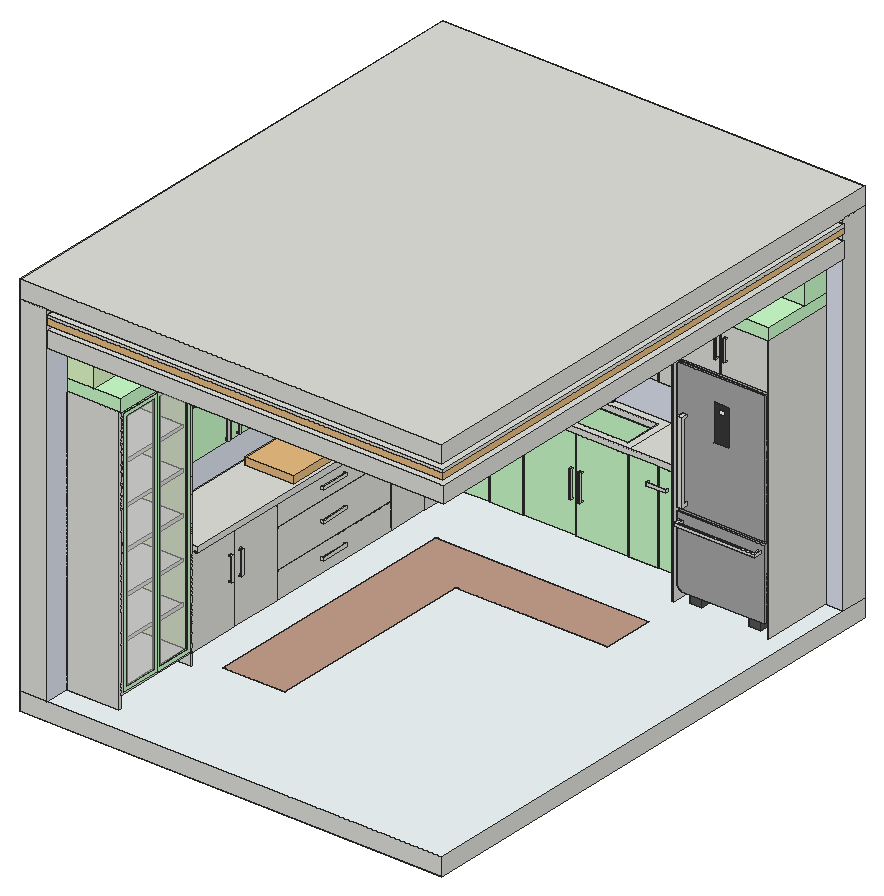
# SketchUp Ruby script. Lengths in inches.
U = 1.inch
M = Sketchup.active_model
def pt(a) = Geom::Point3d.new(a.map { |v| v * U })
def face(e, loops, mat)
  f = e.add_face(loops[0].map { |a| pt(a) })
  loops[1..].each { |l| e.add_face(l.map { |a| pt(a) }).erase! }
  f.material = f.back_material = mat if mat
  f
end
# faces: each face lists its corners as indices into pts; further lists are holes
def faces(e, pts, list, mat = nil) = list.each { |f| face(e, (f[0].is_a?(Array) ? f : [f]).map { |l| l.map { |i| pts[i] } }, mat) }
# xy, xz, yz: faces in a plane at the given z, y or x. An outline is a flat list of corners, or four numbers for a rectangle; further outlines are holes
def ring(l) = l.size == 4 ? [[l[0], l[1]], [l[2], l[1]], [l[2], l[3]], [l[0], l[3]]] : l.each_slice(2).to_a
def flat(e, list, mat, &to3) = list.each { |f| face(e, (f[0].is_a?(Array) ? f : [f]).map { |l| ring(l).map { |u, v| to3.(u, v) } }, mat) }
def xy(e, z, list, mat = nil) = flat(e, list, mat) { |x, y| [x, y, z] }
def xz(e, y, list, mat = nil) = flat(e, list, mat) { |x, z| [x, y, z] }
def yz(e, x, list, mat = nil) = flat(e, list, mat) { |y, z| [x, y, z] }
def lines(e, pts, list) = list.each { |a, b| e.add_line(pt(pts[a]), pt(pts[b])) }
# prism: a flat outline (further loops are holes) pulled along v
def prism(e, loops, v, mat = nil)
  f = face(e, loops, mat); d = Geom::Vector3d.new(v.map { |x| x * U })
  f.pushpull(f.normal.samedirection?(d) ? d.length : -d.length)
end
def box(e, o, s, mat = nil) = prism(e, [[o, [o[0] + s[0], o[1], o[2]], [o[0] + s[0], o[1] + s[1], o[2]], [o[0], o[1] + s[1], o[2]]]], [0, 0, s[2]], mat)
def at(x, y, z, deg = 0) = Geom::Transformation.translation(pt([x, y, z])) * Geom::Transformation.rotation(ORIGIN, Z_AXIS, deg.degrees)
def axes(o, x, y, z) = Geom::Transformation.new([*x, 0, *y, 0, *z, 0, *pt(o).to_a, 1])
def part(name) = M.definitions.add(name)
# library, detail: a bought-in or finely detailed component or shape, given as its bounding box
def library(name, o, s) = part(name).tap { |d| box(d.entities, o, s) }
def detail(e, o, s) = box(e.add_group.entities, o, s)
def put(e, d, t, mat = nil) = e.add_instance(d, t).tap { |i| i.material = mat if mat }
def group(e, t, mat = nil) = e.add_group.tap { |g| g.transformation = t; g.material = mat if mat }.entities
root = M.entities
M.materials.add("[Color E01]").color = [255, 255, 204]
M.materials.add("[Color E04]").color = [255, 255, 50]
M.materials.add("[Color E05]").color = [255, 255, 0]
M.materials.add("[Color F01]").color = [229, 255, 204]
M.materials.add("[Color G01]").color = [204, 255, 204]
M.materials.add("[Color M00]").color = [255, 255, 255]
M.materials.add("[Color M03]").color = [170, 170, 170]
M.materials.add("[Color M06]").color = [86, 86, 86]
M.materials.add("[Color M07]").color = [58, 58, 58]
M.materials.add("[Color M08]").color = [30, 30, 30]
M.materials.add("[Color M09]").color = [0, 0, 0]
M.materials.add("[Marble Carrara Floor Tile]").color = [225, 230, 242]
M.materials.add("[Translucent Glass Gray]").color = [232, 232, 232]
M.materials["[Translucent Glass Gray]"].alpha = 0.5
M.materials.add("[Translucent Glass Gray]1").color = [219, 219, 219]
M.materials["[Translucent Glass Gray]1"].alpha = 0.5
M.materials.add("[Upholstery Striped Multi-Colored]").color = [198, 159, 140]
M.materials.add("[White Subway Tile]").color = [243, 252, 253]
c1 = part("Group\#6")
box(c1.entities,[0,0,0],[17,26,1])
c2 = library("Group\#43",[0,0,0],[16.5,36,2.3125])
c3 = part("Group\#46")
prism(c3.entities,[[[0,1,0],[0,1,0.4],[0.8,1,0.4],[0.8,1,9.6],[0,1,9.6],[0,1,10],[1.2,1,10],[1.2,1,0]]],[0,-1,0])
c4 = part("Group\#47")
prism(c4.entities,[[[0,0,6.4375],[0,0,6.1],[0.66,0,6.1],[0.66,0,0.34],[0,0,0.34],[0,0,0],[1,0,0],[1,0,6.4375]]],[0,0.6875,0])
c5 = part("Group\#49")
prism(c5.entities,[[[0.875,0.31,9],[0.875,1,9],[0.875,1,9.3125],[0.875,0,9.3125],[0.875,0,0],[0.875,1,0],[0.875,1,0.31],[0.875,0.31,0.31]]],[-0.875,0,0])
c6 = part("Group\#50")
prism(c6.entities,[[[6.64,1,0],[6.9375,1,0],[6.9375,0,0],[0,0,0],[0,1,0],[0.3,1,0],[0.3,0.3,0],[6.64,0.3,0]]],[0,0,0.9375])
c7 = part("Group\#51")
prism(c7.entities,[[[0.6875,1,6.95],[0.6875,1,7.25],[0.6875,0,7.25],[0.6875,0,0],[0.6875,1,0],[0.6875,1,0.3],[0.6875,0.3,0.3],[0.6875,0.3,6.95]]],[-0.6875,0,0])
c8 = part("Group\#52")
prism(c8.entities,[[[0,0.5,0],[0,0.5,0.29],[0.8,0.5,0.29],[0.8,0.5,6.98],[0,0.5,6.98],[0,0.5,7.28],[1.2,0.5,7.28],[1.2,0.5,0]]],[0,-0.5,0])
c9 = library("Group\#56",[0,0,0],[135,171,2])
c10 = part("Group\#63")
detail(c10.entities,[0,0,0],[2,2,1.9375])
box(root,[24.44,95.55,73.22],[0.1,9.82,0.69])
xy(root,6,[[34.24,44.3,34.24,134.73,107.05,134.73,107.05,117.05,55.37,117.05,55.37,44.3]])
xy(root,6.01,[[34.24,44.3,55.37,44.3,55.37,117.05,107.05,117.05,107.05,134.73,34.24,134.73]],"[Upholstery Striped Multi-Colored]")
xz(root,44.3,[[34.24,6,55.37,6.01]])
xz(root,117.05,[[55.37,6,107.05,6.01]])
xz(root,134.73,[[34.24,6,107.05,6.01]])
xz(root,147.3,[[121.27,68.89,122.52,70.08]],"[Color M00]")
xz(root,152.9,[[50.8,68.5,66.65,83.5],[67.65,68.5,83.5,83.5]],"[Translucent Glass Gray]")
yz(root,27.5,[[11.5,12.1,23.5,95.05]],"[Translucent Glass Gray]")
yz(root,34.24,[[44.3,6,134.73,6.01]])
yz(root,55.37,[[44.3,6,117.05,6.01]])
yz(root,107.05,[[117.05,6,134.73,6.01]])
p = [[27.5,25.5,95.05],[27,37.5,95.05],[27,37.5,12.1],[27.5,25.5,12.1],[25,106.3,84],[25,94.3,84],
  [10,94.3,84],[10,106.3,84],[11,100.6,45],[27,100.6,45]]
faces(root,p,[[0,1,2,3]],"[Translucent Glass Gray]1")
lines(root,p,[[4,5],[5,6],[6,7],[7,4],[8,9]])
g1 = group(root,at(0,84.5,0))
xy(g1,0,[[0,-84,144,96]])
xy(g1,6,[[0,-84,144,96]],"[White Subway Tile]")
xz(g1,-84,[[0,0,144,6]])
xz(g1,96,[[0,0,144,6]])
yz(g1,0,[[-84,0,96,6]])
yz(g1,144,[[-84,0,96,6]])
g2 = group(root,at(9,171.5,6))
xy(g2,0,[[0,0,135,9]])
xy(g2,120,[[0,0,135,9]])
xz(g2,0,[[0,0,135,120]],"[Marble Carrara Floor Tile]")
xz(g2,9,[[0,0,135,120]])
yz(g2,0,[[0,0,9,120]])
yz(g2,135,[[0,0,9,120]])
g3 = group(root,at(0,84.5,6))
xy(g3,0,[[0,-84,9,96]])
xy(g3,120,[[0,-84,9,96]])
xz(g3,-84,[[0,0,9,120]])
xz(g3,96,[[0,0,9,120]])
yz(g3,0,[[-84,0,96,120]])
yz(g3,9,[[-84,0,96,120]],"[Marble Carrara Floor Tile]")
g4 = group(root,at(9,9.5,6),"[Color G01]")
box(g4,[0,30.5,0],[10,131.5,4])
g5 = group(root,at(9,39.5,6))
box(g5,[0,0,0],[18,0.5,91.15])
g6 = group(root,at(9,9.5,6),"[Color G01]")
box(g6,[0,0,0],[12,30,4])
g7 = group(root,at(9,9,6))
box(g7,[0,0,0],[18,0.5,91.15])
g8 = group(root,at(9,40,10))
xy(g8,0,[[0,0,0,36,18,36,18,18.15,17.7,18.15,17.7,17.85,18,17.85,18,0],[0,36,18,36.6],[0,36.6,18,84.6],[0,84.6,18,84.9],[0,84.9,0,131.5,18,131.5,18,99.5,17.7,99.5,17.7,98.9,18,98.9,18,84.9]])
xy(g8,9,[[14.4,36.6,18,84.6]])
xy(g8,9.3,[[14.4,36.6,18,84.6]])
xy(g8,22,[[14.4,36.6,18,84.6]])
xy(g8,22.3,[[14.4,36.6,18,84.6]])
xy(g8,31,[[0,0,18,0,18,17.85,17.7,17.85,17.7,18.15,18,18.15,18,36,0,36],[0,36,18,36.6],[0,36.6,18,84.6],[0,84.6,18,84.9],[0,84.9,18,84.9,18,98.9,17.7,98.9,17.7,99.5,18,99.5,18,131.5,0,131.5]])
xz(g8,0,[[0,0,18,31]])
xz(g8,17.85,[[17.7,0,18,31]])
xz(g8,18.15,[[17.7,0,18,31]])
xz(g8,36,[[0,0,18,31]])
xz(g8,36.6,[[0,0,0,31,18,31,18,22.3,14.4,22.3,14.4,22,18,22,18,9.3,14.4,9.3,14.4,9,18,9,18,0],[14.4,9,18,9.3],[14.4,22,18,22.3]])
xz(g8,84.6,[[0,0,0,31,18,31,18,22.3,14.4,22.3,14.4,22,18,22,18,9.3,14.4,9.3,14.4,9,18,9,18,0],[14.4,9,18,9.3],[14.4,22,18,22.3]])
xz(g8,84.9,[[0,0,18,31]])
xz(g8,98.9,[[17.7,0,18,31]])
xz(g8,99.5,[[17.7,0,18,31]])
xz(g8,131.5,[[0,0,18,31]])
yz(g8,0,[[0,0,36,31],[36,0,36.6,31],[36.6,0,84.6,31],[84.6,0,84.9,31],[84.9,0,131.5,31]])
yz(g8,14.4,[[36.6,9,84.6,9.3],[36.6,22,84.6,22.3]])
yz(g8,17.7,[[17.85,0,18.15,31],[98.9,0,99.5,31]])
yz(g8,18,[[0,0,17.85,31],[18.15,0,36,31],[36,0,36.6,31],[36.6,0,84.6,9],[84.6,0,84.9,31],
  [84.9,0,98.9,31],[99.5,0,113.5,31],[113.5,0,131.5,31],[36.6,9.3,84.6,22],[36.6,22.3,84.6,31]])
g9 = group(root,at(9,40,41))
prism(g9,[[[0,131.5,0],[0,131.5,2],[20,131.5,2],[20,131.5,0],[19.3,131.5,0],[19.3,131.5,0.3],[19,131.5,0.3],[19,131.5,0]]],[0,-131.5,0])
g10 = group(root,at(9,9.5,10))
g11 = group(g10,at(0,0,0))
g12 = group(g11,at(18,1,1.05),"[Color G01]")
xy(g12,0,[[0,0,0,28,0.5,28,0.5,14.15,0.2,14.15,0.2,13.85,0.5,13.85,0.5,0]])
xy(g12,1.05,[[0,1,0.5,13],[0,15,0.5,27]])
xy(g12,84,[[0,1,0.5,13],[0,15,0.5,27]])
xy(g12,85.05,[[0,0,0.5,0,0.5,13.85,0.2,13.85,0.2,14.15,0.5,14.15,0.5,28,0,28]])
xz(g12,0,[[0,0,0.5,85.05]])
xz(g12,1,[[0,1.05,0.5,84]])
xz(g12,13,[[0,1.05,0.5,84]])
xz(g12,13.85,[[0.2,0,0.5,85.05]])
xz(g12,14.15,[[0.2,0,0.5,85.05]])
xz(g12,15,[[0,1.05,0.5,84]])
xz(g12,27,[[0,1.05,0.5,84]])
xz(g12,28,[[0,0,0.5,85.05]])
yz(g12,0,[[[0,0,28,85.05],[15,1.05,27,84],[1,1.05,13,84]]])
yz(g12,0.2,[[13.85,0,14.15,85.05]])
yz(g12,0.5,[[[0,0,13.85,85.05],[1,1.05,13,84]],[[14.15,0,28,85.05],[15,1.05,27,84]]])
g13 = group(g11,at(0,0,0))
put(g13,c1,axes([0,2,69.3],[1,0,0],[0,1,0],[0,0,1.05]))
put(g13,c1,axes([0,2,42],[1,0,0],[0,1,0],[0,0,1.05]))
put(g13,c1,axes([0,2,55.65],[1,0,0],[0,1,0],[0,0,1.05]))
g14 = group(g13,at(0,0,0))
g15 = group(g14,at(0,0,0))
xy(g15,0,[[0,0,18,30]])
xy(g15,2.1,[[0.1,2,18,28]])
xy(g15,2.1,[[0,2,0.1,28]],"[Color F01]")
xy(g15,85.05,[[0.1,2,18,28]])
xy(g15,85.05,[[0,2,0.1,28]],"[Color F01]")
xy(g15,87.15,[[0,0,18,30]])
xz(g15,0,[[0,0,18,87.15]])
xz(g15,2,[[0.1,2.1,18,85.05]])
xz(g15,2,[[0,2.1,0.1,85.05]],"[Color F01]")
xz(g15,28,[[0,2.1,0.1,85.05],[0.1,2.1,18,85.05]],"[Color F01]")
xz(g15,30,[[0,0,18,87.15]])
yz(g15,0,[[[0,0,30,87.15],[2,2.1,28,85.05]]])
yz(g15,0.1,[[2,2.1,28,85.05]],"[Color F01]")
yz(g15,18,[[[0,0,30,87.15],[2,2.1,28,85.05]]])
put(g13,c1,axes([0,2,14.7],[1,0,0],[0,1,0],[0,0,1.05]))
put(g13,c1,axes([0,2,28.35],[1,0,0],[0,1,0],[0,0,1.05]))
g16 = group(root,at(9,124.3,67),"[Color G01]")
xy(g16,0,[[0,0,17,0.3],[0,0.3,0,29.2,17,29.2,17,14.9,16.7,14.9,16.7,14.6,17,14.6,17,0.3],[0,29.2,17,47.2]])
xy(g16,18,[[0,0,17,0.3],[0,0.3,17,0.3,17,14.6,16.7,14.6,16.7,14.9,17,14.9,17,29.2,0,29.2],[0,29.2,17,47.2]])
xz(g16,0,[[0,0,17,18]])
xz(g16,0.3,[[0,0,17,18]])
xz(g16,14.6,[[16.7,0,17,18]])
xz(g16,14.9,[[16.7,0,17,18]])
xz(g16,29.2,[[0,0,17,18]])
xz(g16,47.2,[[0,0,17,18]])
yz(g16,0,[[0,0,0.3,18],[0.3,0,29.2,18],[29.2,0,47.2,18]])
yz(g16,16.7,[[14.6,0,14.9,18]])
yz(g16,17,[[0,0,0.3,18],[0.3,0,14.6,18],[14.9,0,29.2,18],[29.2,0,47.2,18]])
g17 = group(root,at(9,40,67),"[Color G01]")
xy(g17,0,[[0,0,0,36,17,36,17,18.15,16.7,18.15,16.7,17.85,17,17.85,17,0],[0,36,17,36.3]])
xy(g17,18,[[0,0,17,0,17,17.85,16.7,17.85,16.7,18.15,17,18.15,17,36,0,36],[0,36,17,36.3]])
xz(g17,0,[[0,0,17,18]])
xz(g17,17.85,[[16.7,0,17,18]])
xz(g17,18.15,[[16.7,0,17,18]])
xz(g17,36,[[0,0,17,18]])
xz(g17,36.3,[[0,0,17,18]])
yz(g17,0,[[0,0,36,18],[36,0,36.3,18]])
yz(g17,16.7,[[17.85,0,18.15,18]])
yz(g17,17,[[0,0,17.85,18],[18.15,0,36,18],[36,0,36.3,18]])
g18 = group(root,at(9,76.3,84))
prism(g18,[[[0,0,0],[0,48,0],[16.7,48,0],[16.7,0,0]],[[16,18,0],[16,30,0],[1,30,0],[1,18,0]]],[0,0,1])
g19 = group(root,at(9,40,85))
xy(g19,0,[[0,0,0,36,18.5,36,18.5,18.15,18.2,18.15,18.2,17.85,18.5,17.85,18.5,0],[0,36,18.5,36.6],[[0,36.6,0,83.85,18.5,83.85,18.5,60.375,18.2,60.375,18.2,60.08,18.5,60.08,18.5,36.6],[1,54.23,16,66.23]],[0,83.85,18.5,84.3],[0,84.3,0,113.5,18.5,113.5,18.5,99.05,18.2,99.05,18.2,98.75,18.5,98.75,18.5,84.3],
  [0,113.5,18.5,131.5]])
xy(g19,12.15,[[0,0,18.5,0,18.5,17.85,18.2,17.85,18.2,18.15,18.5,18.15,18.5,36,0,36],[0,36,18.5,36.6],[[0,36.6,18.5,36.6,18.5,60.08,18.2,60.08,18.2,60.375,18.5,60.375,18.5,83.85,0,83.85],[1,54.23,16,66.23]],[0,83.85,18.5,84.3],[0,84.3,18.5,84.3,18.5,98.75,18.2,98.75,18.2,99.05,18.5,99.05,18.5,113.5,0,113.5],
  [0,113.5,18.5,131.5]])
xz(g19,0,[[0,0,18.5,12.15]])
xz(g19,17.85,[[18.2,0,18.5,12.15]])
xz(g19,18.15,[[18.2,0,18.5,12.15]])
xz(g19,36,[[0,0,18.5,12.15]])
xz(g19,36.6,[[0,0,18.5,12.15]])
xz(g19,54.23,[[1,0,16,12.15]])
xz(g19,60.08,[[18.2,0,18.5,12.15]])
xz(g19,60.375,[[18.2,0,18.5,12.15]])
xz(g19,66.23,[[1,0,16,12.15]])
xz(g19,83.85,[[0,0,18.5,12.15]])
xz(g19,84.3,[[0,0,18.5,12.15]])
xz(g19,98.75,[[18.2,0,18.5,12.15]])
xz(g19,99.05,[[18.2,0,18.5,12.15]])
xz(g19,113.5,[[0,0,18.5,12.15]])
xz(g19,131.5,[[0,0,18.5,12.15]])
yz(g19,0,[[0,0,36,12.15],[36,0,36.6,12.15],[36.6,0,83.85,12.15],[83.85,0,84.3,12.15],[84.3,0,113.5,12.15],
  [113.5,0,131.5,12.15]])
yz(g19,1,[[54.23,0,66.23,12.15]])
yz(g19,16,[[54.23,0,66.23,12.15]])
yz(g19,18.2,[[17.85,0,18.15,12.15],[60.08,0,60.375,12.15],[98.75,0,99.05,12.15]])
yz(g19,18.5,[[0,0,17.85,12.15],[18.15,0,36,12.15],[36,0,36.6,12.15],[36.6,0,60.08,12.15],[60.375,0,83.85,12.15],
  [83.85,0,84.3,12.15],[84.3,0,98.75,12.15],[99.05,0,113.5,12.15],[113.5,0,131.5,12.15]])
g20 = group(root,at(9,9,97.15))
xy(g20,0,[[0,0,18.5,162.5]])
xy(g20,4,[[0,0,9.25,29.15],[0,29.15,9.25,67.3],[0,67.3,9.25,115.3],[0,115.3,9.25,144.5],[0,144.5,9.25,162.5]])
xy(g20,4,[[9.25,0,18.5,162.5]],"[Color G01]")
xy(g20,16.85,[[0,0,9.25,29.15],[0,67.3,9.25,115.3],[0,115.3,9.25,144.5],[0,144.5,9.25,162.5]],"[Color F01]")
xy(g20,16.85,[[0,29.15,9.25,67.3]],"[Color G01]")
xz(g20,0,[[0,4,9.25,16.85]],"[Color F01]")
xz(g20,0,[[0,0,18.5,4]],"[Color G01]")
xz(g20,29.15,[[0,4,9.25,16.85]])
xz(g20,67.3,[[0,4,9.25,16.85]])
xz(g20,115.3,[[0,4,9.25,16.85]])
xz(g20,144.5,[[0,4,9.25,16.85]])
xz(g20,162.5,[[0,0,18.5,4],[0,4,9.25,16.85]])
yz(g20,0,[[0,0,162.5,4],[0,4,29.15,16.85],[29.15,4,67.3,16.85],[67.3,4,115.3,16.85],[115.3,4,144.5,16.85],
  [144.5,4,162.5,16.85]])
yz(g20,9.25,[[0,4,29.15,16.85],[67.3,4,115.3,16.85]],"[Color F01]")
yz(g20,9.25,[[29.15,4,67.3,16.85],[115.3,4,144.5,16.85],[144.5,4,162.5,16.85]],"[Color G01]")
yz(g20,18.5,[[0,0,162.5,4]],"[Color G01]")
g21 = group(root,at(9,84.86,67),"[Color M09]")
g22 = group(g21,at(0,0,0))
xy(g22,0,[[0,4,15.44,26.3125],[0,26.3125,15.44,26.88]])
xy(g22,7.5625,[[0,0,15.44,10],[0,10,1.56,20.88],[1.56,10,11,20.88],[11,10,15.44,20.88],[0,20.88,15.44,32.88]])
xy(g22,30.15,[[1.56,10,11,20.88]])
xz(g22,10,[[1.56,7.5625,11,30.15]])
xz(g22,20.88,[[1.56,7.5625,11,30.15]])
yz(g22,0,[[4,0,0,7.5625,32.88,7.5625,26.88,0]])
yz(g22,1.56,[[10,7.5625,20.88,30.15]])
yz(g22,11,[[10,7.5625,20.88,30.15]])
yz(g22,15.44,[[4,0,26.88,0,32.88,7.5625,0,7.5625]])
p = [[15.44,4,0],[15.44,0,7.5625],[0,0,7.5625],[0,4,0],[15.44,32.88,7.5625],[15.44,26.88,0],
  [0,26.88,0],[0,32.88,7.5625]]
faces(g22,p,[[0,1,2,3],[4,5,6,7]])
g23 = group(root,at(19,161.5,6),"[Color G01]")
box(g23,[0,0,0],[86,10,4])
g24 = group(root,at(27,153.5,10),"[Color G01]")
xy(g24,0,[[0,0,0,18,22,18,22,0,10.65,0,10.65,0.3,10.35,0.3,10.35,0],[22,0,22.3,18],[22.3,0,22.3,18,58,18,58,0,40.3,0,40.3,0.3,40,0.3,40,0],[58,0,58.3,18],[58.3,0,58.3,18,78,18,78,0,68.3,0,68.3,0.3,68,0.3,68,0]])
xy(g24,7.5,[[23.8,1.5,56.5,15.25]])
xy(g24,31,[[0,0,10.35,0,10.35,0.3,10.65,0.3,10.65,0,22,0,22,18,0,18],[22,0,22.3,18],[[22.3,0,40,0,40,0.3,40.3,0.3,40.3,0,58,0,58,18,22.3,18],[23.8,1.5,56.5,15.25]],[58,0,58.3,18],[58.3,0,68,0,68,0.3,68.3,0.3,68.3,0,78,0,78,18,58.3,18]])
xz(g24,0,[[0,0,10.35,31],[10.65,0,22,31],[22,0,22.3,31],[22.3,0,40,31],[40.3,0,58,31],
  [58,0,58.3,31],[58.3,0,68,31],[68.3,0,78,31]])
xz(g24,0.3,[[10.35,0,10.65,31],[40,0,40.3,31],[68,0,68.3,31]])
xz(g24,1.5,[[23.8,7.5,56.5,31]])
xz(g24,15.25,[[23.8,7.5,56.5,31]])
xz(g24,18,[[0,0,22,31],[22,0,22.3,31],[22.3,0,58,31],[58,0,58.3,31],[58.3,0,78,31]])
yz(g24,0,[[0,0,18,31]])
yz(g24,10.35,[[0,0,0.3,31]])
yz(g24,10.65,[[0,0,0.3,31]])
yz(g24,22,[[0,0,18,31]])
yz(g24,22.3,[[0,0,18,31]])
yz(g24,23.8,[[1.5,7.5,15.25,31]])
yz(g24,40,[[0,0,0.3,31]])
yz(g24,40.3,[[0,0,0.3,31]])
yz(g24,56.5,[[1.5,7.5,15.25,31]])
yz(g24,58,[[0,0,18,31]])
yz(g24,58.3,[[0,0,18,31]])
yz(g24,68,[[0,0,0.3,31]])
yz(g24,68.3,[[0,0,0.3,31]])
yz(g24,78,[[0,0,18,31]])
g25 = group(root,at(105,153.5,10))
box(g25,[0,-6.2,-4],[0.5,24.2,91.15])
g26 = group(root,at(26,153.5,67))
xy(g26,0,[[23.3,-0.3,59,17.9],[0,0,0,18,23,18,23,0,11.65,0,11.65,0.3,11.35,0.3,11.35,0],[23,0,23.3,18],[59,0,59.3,18],[59.3,0,59.3,18,79,18,79,0,69.3,0,69.3,0.3,69,0.3,69,0]])
xy(g26,1,[[24.3,-0.3,58,0]])
xy(g26,5,[[23.3,2.9,59,17.9]])
xy(g26,5.5,[[23.3,2.9,59,17.9]])
xy(g26,10.5,[[23.3,2.9,59,17.9]])
xy(g26,11,[[23.3,2.9,59,17.9]])
xy(g26,17,[[24.3,-0.3,58,0]])
xy(g26,18,[[23.3,-0.3,59,17.9],[0,0,11.35,0,11.35,0.3,11.65,0.3,11.65,0,23,0,23,18,0,18],[23,0,23.3,18],[59,0,59.3,18],[59.3,0,69,0,69,0.3,69.3,0.3,69.3,0,79,0,79,18,59.3,18]])
xz(g26,-0.3,[[[23.3,0,59,18],[24.3,1,58,17]]])
xz(g26,0,[[0,0,11.35,18],[11.65,0,23,18],[23,0,23.3,18],[59,0,59.3,18],[59.3,0,69,18],
  [69.3,0,79,18]])
xz(g26,0.3,[[11.35,0,11.65,18],[69,0,69.3,18]])
xz(g26,2.9,[[23.3,5,59,5.5],[23.3,10.5,59,11]])
xz(g26,17.9,[[23.3,0,59,5],[23.3,5.5,59,10.5],[23.3,11,59,18]])
xz(g26,18,[[0,0,23,18],[23,0,23.3,18],[59,0,59.3,18],[59.3,0,79,18]])
yz(g26,0,[[0,0,18,18]])
yz(g26,11.35,[[0,0,0.3,18]])
yz(g26,11.65,[[0,0,0.3,18]])
yz(g26,23,[[0,0,18,18]])
yz(g26,23.3,[[-0.3,0,0,18],[0,0,17.9,0,17.9,5,2.9,5,2.9,5.5,17.9,5.5,17.9,10.5,2.9,10.5,2.9,11,17.9,11,17.9,18,0,18],[17.9,0,18,0,18,18,17.9,18,17.9,11,2.9,11,2.9,10.5,17.9,10.5,17.9,5.5,2.9,5.5,2.9,5,17.9,5]])
yz(g26,24.3,[[-0.3,1,0,17]])
yz(g26,58,[[-0.3,1,0,17]])
yz(g26,59,[[-0.3,0,0,18],[0,0,17.9,0,17.9,5,2.9,5,2.9,5.5,17.9,5.5,17.9,10.5,2.9,10.5,2.9,11,17.9,11,17.9,18,0,18],[17.9,0,18,0,18,18,17.9,18,17.9,11,2.9,11,2.9,10.5,17.9,10.5,17.9,5.5,2.9,5.5,2.9,5,17.9,5]])
yz(g26,59.3,[[0,0,18,18]])
yz(g26,69,[[0,0,0.3,18]])
yz(g26,69.3,[[0,0,0.3,18]])
yz(g26,79,[[0,0,18,18]])
g27 = group(root,at(50.3,152.9,68))
prism(g27,[[[33.7,0,16],[0,0,16],[0,0,0],[33.7,0,0]],[[0.5,0,15.5],[16.35,0,15.5],[16.35,0,0.5],[0.5,0,0.5]],[[17.35,0,15.5],[33.2,0,15.5],[33.2,0,0.5],[17.35,0,0.5]]],[0,0.3,0])
g28 = group(root,at(27.5,152.3,85))
xy(g28,0,[[0,0,0,19.2,21.5,19.2,21.5,0,10.9,0,10.9,0.3,10.6,0.3,10.6,0],[21.5,0,21.8,19.2],[21.8,0,21.8,19.2,57.5,19.2,57.5,0,39.8,0,39.8,0.3,39.5,0.3,39.5,0],[57.5,0,57.8,19.2],[57.8,0,57.8,19.2,77.5,19.2,77.5,0,67.8,0,67.8,0.3,67.5,0.3,67.5,0]])
xy(g28,12.15,[[0,0,10.6,0,10.6,0.3,10.9,0.3,10.9,0,21.5,0,21.5,19.2,0,19.2],[21.5,0,21.8,19.2],[21.8,0,39.5,0,39.5,0.3,39.8,0.3,39.8,0,57.5,0,57.5,19.2,21.8,19.2],[57.5,0,57.8,19.2],[57.8,0,67.5,0,67.5,0.3,67.8,0.3,67.8,0,77.5,0,77.5,19.2,57.8,19.2]])
xz(g28,0,[[0,0,10.6,12.15],[10.9,0,21.5,12.15],[21.5,0,21.8,12.15],[21.8,0,39.5,12.15],[39.8,0,57.5,12.15],
  [57.5,0,57.8,12.15],[57.8,0,67.5,12.15],[67.8,0,77.5,12.15]])
xz(g28,0.3,[[10.6,0,10.9,12.15],[39.5,0,39.8,12.15],[67.5,0,67.8,12.15]])
xz(g28,19.2,[[0,0,21.5,12.15],[21.5,0,21.8,12.15],[21.8,0,57.5,12.15],[57.5,0,57.8,12.15],[57.8,0,77.5,12.15]])
yz(g28,0,[[0,0,19.2,12.15]])
yz(g28,10.6,[[0,0,0.3,12.15]])
yz(g28,10.9,[[0,0,0.3,12.15]])
yz(g28,21.5,[[0,0,19.2,12.15]])
yz(g28,21.8,[[0,0,19.2,12.15]])
yz(g28,39.5,[[0,0,0.3,12.15]])
yz(g28,39.8,[[0,0,0.3,12.15]])
yz(g28,57.5,[[0,0,19.2,12.15]])
yz(g28,57.8,[[0,0,19.2,12.15]])
yz(g28,67.5,[[0,0,0.3,12.15]])
yz(g28,67.8,[[0,0,0.3,12.15]])
yz(g28,77.5,[[0,0,19.2,12.15]])
g29 = group(root,at(27.5,152.3,97.15),"[Color G01]")
box(g29,[0,0,0],[77.5,19.2,4])
g30 = group(root,at(137.5,149.3,6))
box(g30,[0,-2,0],[0.5,24.2,91.15])
g31 = group(root,at(131.5,149.3,6),"[Color M06]")
box(g31,[-2,0,0],[4,22.2,4])
g32 = group(root,at(109.5,149.3,6),"[Color M06]")
box(g32,[0,0,0],[4,26.2,4])
g33 = group(root,at(106.5,147.3,10),"[Color M03]")
g34 = group(g33,at(0,1,0))
box(g34,[0,-0.1,0],[30,23.3,69.75])
g35 = group(g33,at(0,0,0))
xy(g35,0,[[1.66,0,30,1]])
xy(g35,24.01,[[0,0,30,1]])
xy(g35,25.21,[[0,0,30,1]])
xy(g35,69.75,[[1.21,0,30,1]])
xz(g35,0,[[1.66,0,1.41,0.13,1.18,0.27,0.97,0.43,0.77,0.6,0.6,0.79,0.44,0.99,0.31,1.19,0.2,1.41,0.11,1.63,0.05,1.86,0.01,2.09,0,2.32,0,24.01,30,24.01,30,0],[[0,25.21,0,68.625,0.01,68.76,0.04,68.89,0.09,69.02,0.16,69.14,0.24,69.26,0.34,69.37,0.46,69.46,0.59,69.55,0.73,69.62,0.88,69.68,1.04,69.72,1.21,69.75,30,69.75,30,25.21],[12.66,49.36,18.29,62.05]]])
xz(g35,0,[[12.66,49.36,18.29,62.05]],"[Color M07]")
xz(g35,1,[[0,0,0,2.32,0.01,2.09,0.05,1.86,0.11,1.63,0.2,1.41,0.31,1.19,0.44,0.99,0.6,0.79,0.77,0.6,0.97,0.43,1.18,0.27,1.41,0.13,1.66,0],[0,24.01,30,25.21],[0,68.625,0,69.75,1.21,69.75,1.04,69.72,0.88,69.68,0.73,69.62,0.59,69.55,0.46,69.46,0.34,69.37,0.24,69.26,0.16,69.14,0.09,69.02,0.04,68.89,0.01,68.76]])
yz(g35,0,[[0,2.32,1,24.01],[0,25.21,1,68.625]])
yz(g35,30,[[0,0,1,24.01],[0,25.21,1,69.75]])
p = [[1.66,1,0],[1.41,1,0.13],[1.41,0,0.13],[1.66,0,0],[1.18,1,0.27],[1.18,0,0.27],
  [0.97,1,0.43],[0.97,0,0.43],[0.77,1,0.6],[0.77,0,0.6],[0.6,1,0.79],[0.6,0,0.79],
  [0.44,1,0.99],[0.44,0,0.99],[0.31,1,1.19],[0.31,0,1.19],[0.2,1,1.41],[0.2,0,1.41],
  [0.11,1,1.63],[0.11,0,1.63],[0.05,1,1.86],[0.05,0,1.86],[0.01,1,2.09],[0.01,0,2.09],
  [0,1,2.32],[0,0,2.32],[0,1,68.625],[0.01,1,68.76],[0.01,0,68.76],[0,0,68.625],
  [0.04,1,68.89],[0.04,0,68.89],[0.09,1,69.02],[0.09,0,69.02],[0.16,1,69.14],[0.16,0,69.14],
  [0.24,1,69.26],[0.24,0,69.26],[0.34,1,69.37],[0.34,0,69.37],[0.46,1,69.46],[0.46,0,69.46],
  [0.59,1,69.55],[0.59,0,69.55],[0.73,1,69.62],[0.73,0,69.62],[0.88,1,69.68],[0.88,0,69.68],
  [1.04,1,69.72],[1.04,0,69.72],[1.21,1,69.75],[1.21,0,69.75]]
faces(g35,p,[[0,1,2,3],[1,4,5,2],[4,6,7,5],[6,8,9,7],[8,10,11,9],[10,12,13,11],[12,14,15,13],[14,16,17,15],
  [16,18,19,17],[18,20,21,19],[20,22,23,21],[22,24,25,23],[26,27,28,29],[27,30,31,28],[30,32,33,31],[32,34,35,33],
  [34,36,37,35],[36,38,39,37],[38,40,41,39],[40,42,43,41],[42,44,45,43],[44,46,47,45],[46,48,49,47],[48,50,51,49]])
g36 = group(root,at(105.5,147.3,81.12))
prism(g36,[[[0,24.2,0],[32,24.2,0],[32,0,0],[16.15,0,0],[16.15,0.3,0],[15.85,0.3,0],[15.85,0,0],[0,0,0]]],[0,0,16.03])
g37 = group(root,at(105,147.2,97.15),"[Color G01]")
box(g37,[0,0,0],[33,24.3,4])
g38 = group(root,at(18.25,162.5,101.15))
xy(g38,0,[[0,0,86.75,9],[86.75,0,94.75,9],[94.75,0,102.75,9],[102.75,0,110.75,9],[111.05,0,119.75,9],
  [110.75,0.3,111.05,9]])
xy(g38,12.85,[[110.75,0.3,111.05,9]])
xy(g38,12.85,[[0,0,86.75,9],[94.75,0,102.75,9],[102.75,0,110.75,9]],"[Color F01]")
xy(g38,12.85,[[86.75,0,94.75,9],[111.05,0,119.75,9]],"[Color G01]")
xz(g38,0,[[0,0,86.75,12.85],[94.75,0,102.75,12.85],[102.75,0,110.75,12.85]],"[Color F01]")
xz(g38,0,[[86.75,0,94.75,12.85],[111.05,0,119.75,12.85]],"[Color G01]")
xz(g38,0.3,[[110.75,0,111.05,12.85]])
xz(g38,9,[[0,0,86.75,12.85],[86.75,0,94.75,12.85],[94.75,0,102.75,12.85],[102.75,0,110.75,12.85],[110.75,0,111.05,12.85],
  [111.05,0,119.75,12.85]])
yz(g38,0,[[0,0,9,12.85]])
yz(g38,86.75,[[0,0,9,12.85]])
yz(g38,94.75,[[0,0,9,12.85]])
yz(g38,102.75,[[0,0,9,12.85]])
yz(g38,110.75,[[0,0,0.3,12.85],[0.3,0,9,12.85]])
yz(g38,111.05,[[0,0,0.3,12.85],[0.3,0,9,12.85]])
yz(g38,119.75,[[0,0,9,12.85]],"[Color G01]")
put(root,c2,at(11,82.6,43),"[Color M08]")
g39 = group(root,at(107.98,144.3,37))
prism(g39,[[[0.625,3,27.8125],[0.625,3,26.99],[0.625,1.38,26.99],[0.625,1.38,1.13],[0.625,3,1.13],[0.625,3,0],[0.625,0.625,0],[0.625,0.625,27.8125]]],[1.5,0,0])
g40 = group(root,at(107.31,144.3,33.22))
prism(g40,[[[26.99,3,-2.3125],[27.8125,3,-2.3125],[27.8125,0.625,-2.3125],[0,0.625,-2.3125],[0,3,-2.3125],[1.13,3,-2.3125],[1.13,1.38,-2.3125],[26.99,1.38,-2.3125]]],[0,0,0.875])
put(root,c3,axes([27,94.54,26.82],[1,0,0],[0,0,-1],[0,1,0]))
put(root,c3,axes([27,94.54,37.01],[1,0,0],[0,0,-1],[0,1,0]))
put(root,c3,axes([27,94.54,15.44],[1,0,0],[0,0,-1],[0,1,0]))
put(root,c4,axes([27.5,56.68,87.52],[1,0,0],[0,1,0],[0,0,0.7]))
put(root,c4,axes([27.5,58.8,87.52],[1,0,0],[0,1,0],[0,0,0.7]))
put(root,c4,axes([27.5,139.61,87.52],[1,0,0],[0,1,0],[0,0,0.7]))
put(root,c4,axes([27.5,137.36,87.52],[1,0,0],[0,1,0],[0,0,0.7]))
put(root,c4,axes([27.5,101.8,87.52],[1,0,0],[0,1,0],[0,0,0.7]))
put(root,c4,axes([27.5,98.3,87.52],[1,0,0],[0,1,0],[0,0,0.7]))
put(root,c5,at(35.23,152.5,20.9375))
put(root,c5,at(38.85,152.5,20.9375))
put(root,c5,at(65.41,152.5,20.9375))
put(root,c5,at(68.54,152.5,20.9375))
put(root,c5,axes([96.83,152.5,72.08],[1,0,0],[0,1,0],[0,0,0.8439]))
put(root,c5,axes([92.58,152.5,72.08],[1,0,0],[0,1,0],[0,0,0.8439]))
put(root,c5,axes([38.65,152.375,71.03],[1,0,0],[0,1,0],[0,0,0.8439]))
put(root,c5,axes([35.14,152.375,71.03],[1,0,0],[0,1,0],[0,0,0.8439]))
put(root,c6,at(91.6875,152.5,34.38))
put(root,c6,at(91.74,151.3,86.7))
put(root,c6,at(63.99,151.3,86.7))
put(root,c6,at(34.99,151.3,86.7))
put(root,c7,at(119.83,146.3,85.7))
put(root,c7,at(122.83,146.3,85.7))
put(root,c8,at(26,55.2,67.97))
put(root,c8,at(26,60.01,67.97))
put(root,c8,at(26,137.2,67.97))
put(root,c8,at(26,140.39,67.97))
g41 = group(root,at(27,55.35,24.85))
prism(g41,[[[0,1,0],[0,1,0.33],[0.8,1,0.33],[0.8,1,7.86],[0,1,7.86],[0,1,8.1875],[1.2,1,8.1875],[1.2,1,0]]],[0,-1,0])
g42 = group(root,at(27,59.79,24.85))
prism(g42,[[[0,1,0],[0,1,0.33],[0.8,1,0.33],[0.8,1,7.86],[0,1,7.86],[0,1,8.1875],[1.2,1,8.1875],[1.2,1,0]]],[0,-1,0])
g43 = group(root,at(27,136.48,24.85))
prism(g43,[[[0,0,8.1875],[0,0,7.86],[0.8,0,7.86],[0.8,0,0.33],[0,0,0.33],[0,0,0],[1.2,0,0],[1.2,0,8.1875]]],[0,1,0])
g44 = group(root,at(27,140.85,24.85))
prism(g44,[[[0,0,8.1875],[0,0,7.86],[0.8,0,7.86],[0.8,0,0.33],[0,0,0.33],[0,0,0],[1.2,0,0],[1.2,0,8.1875]]],[0,1,0])
g45 = group(root,at(9,0,114))
xy(g45,8.5625,[[60.32,87.37,58.52,87.6,56.85,88.3,55.41,89.4,54.31,90.83,53.62,92.51,53.38,94.3,53.62,96.1,54.31,97.77,55.41,99.21,56.85,100.3125,58.52,101,60.32,101.24,62.11,101,63.79,100.3125,65.22,99.21,66.33,97.77,67.02,96.1,67.26,94.3,67.02,92.51,66.33,90.83,65.22,89.4,63.79,88.3,62.11,87.6]],"[Color M09]")
xy(g45,9.5625,[[[0.4375,0,135.4375,171],[60.32,87.37,62.11,87.6,63.79,88.3,65.22,89.4,66.33,90.83,67.02,92.51,67.26,94.3,67.02,96.1,66.33,97.77,65.22,99.21,63.79,100.3125,62.11,101,60.32,101.24,58.52,101,56.85,100.3125,55.41,99.21,54.31,97.77,53.62,96.1,53.38,94.3,53.62,92.51,54.31,90.83,55.41,89.4,56.85,88.3,58.52,87.6]]],"[Color G01]")
xy(g45,10.5625,[[0.4375,0,135.4375,171]])
xz(g45,0,[[0.4375,9.5625,135.4375,10.5625]])
xz(g45,171,[[0.4375,9.5625,135.4375,10.5625]])
yz(g45,0.4375,[[0,9.5625,171,10.5625]])
yz(g45,135.4375,[[0,9.5625,171,10.5625]])
p = [[60.32,87.37,9.5625],[58.52,87.6,9.5625],[58.52,87.6,8.5625],[60.32,87.37,8.5625],[62.11,87.6,9.5625],[62.11,87.6,8.5625],
  [56.85,88.3,9.5625],[56.85,88.3,8.5625],[63.79,88.3,9.5625],[63.79,88.3,8.5625],[55.41,89.4,9.5625],[55.41,89.4,8.5625],
  [65.22,89.4,9.5625],[65.22,89.4,8.5625],[54.31,90.83,9.5625],[54.31,90.83,8.5625],[66.33,90.83,9.5625],[66.33,90.83,8.5625],
  [53.62,92.51,9.5625],[53.62,92.51,8.5625],[67.02,92.51,9.5625],[67.02,92.51,8.5625],[53.38,94.3,9.5625],[53.38,94.3,8.5625],
  [67.26,94.3,9.5625],[67.26,94.3,8.5625],[53.62,96.1,9.5625],[53.62,96.1,8.5625],[67.02,96.1,9.5625],[67.02,96.1,8.5625],
  [54.31,97.77,9.5625],[54.31,97.77,8.5625],[66.33,97.77,9.5625],[66.33,97.77,8.5625],[55.41,99.21,9.5625],[55.41,99.21,8.5625],
  [65.22,99.21,9.5625],[65.22,99.21,8.5625],[56.85,100.3125,9.5625],[56.85,100.3125,8.5625],[63.79,100.3125,9.5625],[63.79,100.3125,8.5625],
  [58.52,101,9.5625],[58.52,101,8.5625],[62.11,101,9.5625],[62.11,101,8.5625],[60.32,101.24,9.5625],[60.32,101.24,8.5625]]
faces(g45,p,[[0,1,2,3],[4,0,3,5],[1,6,7,2],[8,4,5,9],[6,10,11,7],[12,8,9,13],[10,14,15,11],[16,12,13,17],
  [14,18,19,15],[20,16,17,21],[18,22,23,19],[24,20,21,25],[22,26,27,23],[28,24,25,29],[26,30,31,27],[32,28,29,33],
  [30,34,35,31],[36,32,33,37],[34,38,39,35],[40,36,37,41],[38,42,43,39],[44,40,41,45],[42,46,47,43],[46,44,45,47]],"[Color M09]")
g46 = group(g45,at(0,0.5,0))
xy(g46,0,[[[0,0,135.4375,170.5],[10.52,14.58,127.23,152.54]]])
xy(g46,3.5625,[[[10.52,14.58,127.23,152.54],[111.65,15.88,95.56,146.05,12.95,146.05,12.95,66.73],[34.9375,32.91,35.64,33,36.29,33.28,36.86,33.71,37.29,34.27,37.56,34.92,37.65,35.62,37.56,36.32,37.29,36.98,36.86,37.54,36.29,37.97,35.64,38.24,34.9375,38.33,34.24,38.24,33.58,37.97,33.02,37.54,32.59,36.98,32.32,36.32,32.23,35.62,32.32,34.92,32.59,34.27,33.02,33.71,33.58,33.28,34.24,33],[111.2,137.23,111.71,137.33,112.18,137.55,112.58,137.89,112.87,138.33,113.04,138.82,113.08,139.34,112.99,139.85,112.76,140.32,112.42,140.72,111.99,141.01,111.5,141.19,110.98,141.22,110.46,141.13,109.99,140.9,109.6,140.5625,109.3,140.13,109.13,139.64,109.09,139.12,109.19,138.6,109.41,138.13,109.75,137.74,110.18,137.44,110.68,137.27]]])
xy(g46,3.6875,[[[111.2,137.23,110.68,137.27,110.18,137.44,109.75,137.74,109.41,138.13,109.19,138.6,109.09,139.12,109.13,139.64,109.3,140.13,109.6,140.5625,109.99,140.9,110.46,141.13,110.98,141.22,111.5,141.19,111.99,141.01,112.42,140.72,112.76,140.32,112.99,139.85,113.08,139.34,113.04,138.82,112.87,138.33,112.58,137.89,112.18,137.55,111.71,137.33],[111.09,137.6,111.51,137.66,111.9,137.82,112.23,138.08,112.49,138.42,112.66,138.81,112.71,139.23,112.66,139.65,112.49,140.04,112.23,140.375,111.9,140.64,111.51,140.8,111.09,140.85,110.67,140.8,110.27,140.64,109.9375,140.375,109.68,140.04,109.52,139.65,109.46,139.23,109.52,138.81,109.68,138.42,109.9375,138.08,110.27,137.82,110.67,137.66]]],"[Color E05]")
xy(g46,3.75,[[[34.9375,32.91,34.24,33,33.58,33.28,33.02,33.71,32.59,34.27,32.32,34.92,32.23,35.62,32.32,36.32,32.59,36.98,33.02,37.54,33.58,37.97,34.24,38.24,34.9375,38.33,35.64,38.24,36.29,37.97,36.86,37.54,37.29,36.98,37.56,36.32,37.65,35.62,37.56,34.92,37.29,34.27,36.86,33.71,36.29,33.28,35.64,33],[35.15,33.63,35.66,33.76,36.12,34.01,36.49,34.37,36.77,34.8125,36.91,35.3125,36.93,35.83,36.81,36.34,36.56,36.8,36.2,37.18,35.75,37.45,35.25,37.6,34.73,37.61,34.22,37.49,33.76,37.24,33.38,36.88,33.11,36.43,32.96,35.93,32.95,35.41,33.07,34.9,33.32,34.45,33.68,34.07,34.13,33.79,34.63,33.65]]],"[Color E04]")
xy(g46,3.9375,[[111.09,137.6,110.67,137.66,110.27,137.82,109.9375,138.08,109.68,138.42,109.52,138.81,109.46,139.23,109.52,139.65,109.68,140.04,109.9375,140.375,110.27,140.64,110.67,140.8,111.09,140.85,111.51,140.8,111.9,140.64,112.23,140.375,112.49,140.04,112.66,139.65,112.71,139.23,112.66,138.81,112.49,138.42,112.23,138.08,111.9,137.82,111.51,137.66]],"[Color E05]")
xy(g46,4.25,[[35.15,33.63,34.63,33.65,34.13,33.79,33.68,34.07,33.32,34.45,33.07,34.9,32.95,35.41,32.96,35.93,33.11,36.43,33.38,36.88,33.76,37.24,34.22,37.49,34.73,37.61,35.25,37.6,35.75,37.45,36.2,37.18,36.56,36.8,36.81,36.34,36.93,35.83,36.91,35.3125,36.77,34.8125,36.49,34.37,36.12,34.01,35.66,33.76]],"[Color E04]")
xy(g46,5.5625,[[[0,0,135.4375,170.5],[111.65,15.88,12.95,66.73,12.95,146.05,95.56,146.05]]])
xz(g46,0,[[0,0,135.4375,5.5625]])
xz(g46,14.58,[[10.52,0,127.23,3.5625]])
xz(g46,146.05,[[12.95,3.5625,95.56,5.5625]])
xz(g46,152.54,[[10.52,0,127.23,3.5625]])
xz(g46,170.5,[[0,0,135.4375,5.5625]])
yz(g46,0,[[0,0,170.5,5.5625]])
yz(g46,10.52,[[14.58,0,152.54,3.5625]])
yz(g46,12.95,[[66.73,3.5625,146.05,5.5625]])
yz(g46,127.23,[[14.58,0,152.54,3.5625]])
yz(g46,135.4375,[[0,0,170.5,5.5625]])
p = [[12.95,66.73,5.5625],[111.65,15.88,5.5625],[111.65,15.88,3.5625],[12.95,66.73,3.5625],[95.56,146.05,5.5625],[95.56,146.05,3.5625],
  [34.9375,32.91,3.5625],[34.24,33,3.5625],[34.24,33,3.75],[34.9375,32.91,3.75],[35.64,33,3.5625],[35.64,33,3.75],
  [33.58,33.28,3.5625],[33.58,33.28,3.75],[36.29,33.28,3.5625],[36.29,33.28,3.75],[33.02,33.71,3.5625],[33.02,33.71,3.75],
  [36.86,33.71,3.5625],[36.86,33.71,3.75],[32.59,34.27,3.5625],[32.59,34.27,3.75],[37.29,34.27,3.5625],[37.29,34.27,3.75],
  [32.32,34.92,3.5625],[32.32,34.92,3.75],[37.56,34.92,3.5625],[37.56,34.92,3.75],[32.23,35.62,3.5625],[32.23,35.62,3.75],
  [37.65,35.62,3.5625],[37.65,35.62,3.75],[32.32,36.32,3.5625],[32.32,36.32,3.75],[37.56,36.32,3.5625],[37.56,36.32,3.75],
  [32.59,36.98,3.5625],[32.59,36.98,3.75],[37.29,36.98,3.5625],[37.29,36.98,3.75],[33.02,37.54,3.5625],[33.02,37.54,3.75],
  [36.86,37.54,3.5625],[36.86,37.54,3.75],[33.58,37.97,3.5625],[33.58,37.97,3.75],[36.29,37.97,3.5625],[36.29,37.97,3.75],
  [34.24,38.24,3.5625],[34.24,38.24,3.75],[35.64,38.24,3.5625],[35.64,38.24,3.75],[34.9375,38.33,3.5625],[34.9375,38.33,3.75],
  [111.2,137.23,3.5625],[110.68,137.27,3.5625],[110.68,137.27,3.6875],[111.2,137.23,3.6875],[111.71,137.33,3.5625],[111.71,137.33,3.6875],
  [110.18,137.44,3.5625],[110.18,137.44,3.6875],[112.18,137.55,3.5625],[112.18,137.55,3.6875],[109.75,137.74,3.5625],[109.75,137.74,3.6875],
  [112.58,137.89,3.5625],[112.58,137.89,3.6875],[109.41,138.13,3.5625],[109.41,138.13,3.6875],[112.87,138.33,3.5625],[112.87,138.33,3.6875],
  [109.19,138.6,3.5625],[109.19,138.6,3.6875],[113.04,138.82,3.5625],[113.04,138.82,3.6875],[109.09,139.12,3.5625],[109.09,139.12,3.6875],
  [113.08,139.34,3.5625],[113.08,139.34,3.6875],[109.13,139.64,3.5625],[109.13,139.64,3.6875],[112.99,139.85,3.5625],[112.99,139.85,3.6875],
  [109.3,140.13,3.5625],[109.3,140.13,3.6875],[112.76,140.32,3.5625],[112.76,140.32,3.6875],[109.6,140.5625,3.5625],[109.6,140.5625,3.6875],
  [112.42,140.72,3.5625],[112.42,140.72,3.6875],[109.99,140.9,3.5625],[109.99,140.9,3.6875],[111.99,141.01,3.5625],[111.99,141.01,3.6875],
  [110.46,141.13,3.5625],[110.46,141.13,3.6875],[111.5,141.19,3.5625],[111.5,141.19,3.6875],[110.98,141.22,3.5625],[110.98,141.22,3.6875],
  [111.09,137.6,3.9375],[111.09,137.6,3.6875],[110.67,137.66,3.6875],[110.67,137.66,3.9375],[111.51,137.66,3.9375],[111.51,137.66,3.6875],
  [110.27,137.82,3.6875],[110.27,137.82,3.9375],[111.9,137.82,3.9375],[111.9,137.82,3.6875],[109.9375,138.08,3.6875],[109.9375,138.08,3.9375],
  [112.23,138.08,3.9375],[112.23,138.08,3.6875],[109.68,138.42,3.6875],[109.68,138.42,3.9375],[112.49,138.42,3.9375],[112.49,138.42,3.6875],
  [109.52,138.81,3.6875],[109.52,138.81,3.9375],[112.66,138.81,3.9375],[112.66,138.81,3.6875],[109.46,139.23,3.6875],[109.46,139.23,3.9375],
  [112.71,139.23,3.9375],[112.71,139.23,3.6875],[109.52,139.65,3.6875],[109.52,139.65,3.9375],[112.66,139.65,3.9375],[112.66,139.65,3.6875],
  [109.68,140.04,3.6875],[109.68,140.04,3.9375],[112.49,140.04,3.9375],[112.49,140.04,3.6875],[109.9375,140.375,3.6875],[109.9375,140.375,3.9375],
  [112.23,140.375,3.9375],[112.23,140.375,3.6875],[110.27,140.64,3.6875],[110.27,140.64,3.9375],[111.9,140.64,3.9375],[111.9,140.64,3.6875],
  [110.67,140.8,3.6875],[110.67,140.8,3.9375],[111.51,140.8,3.9375],[111.51,140.8,3.6875],[111.09,140.85,3.6875],[111.09,140.85,3.9375],
  [34.63,33.65,4.25],[34.63,33.65,3.75],[34.13,33.79,3.75],[34.13,33.79,4.25],[35.15,33.63,4.25],[35.15,33.63,3.75],
  [35.66,33.76,4.25],[35.66,33.76,3.75],[33.68,34.07,3.75],[33.68,34.07,4.25],[36.12,34.01,4.25],[36.12,34.01,3.75],
  [36.49,34.37,4.25],[36.49,34.37,3.75],[33.32,34.45,3.75],[33.32,34.45,4.25],[33.07,34.9,3.75],[33.07,34.9,4.25],
  [36.77,34.8125,4.25],[36.77,34.8125,3.75],[36.91,35.3125,4.25],[36.91,35.3125,3.75],[32.95,35.41,3.75],[32.95,35.41,4.25],
  [36.93,35.83,4.25],[36.93,35.83,3.75],[32.96,35.93,3.75],[32.96,35.93,4.25],[36.81,36.34,4.25],[36.81,36.34,3.75],
  [33.11,36.43,3.75],[33.11,36.43,4.25],[36.56,36.8,4.25],[36.56,36.8,3.75],[33.38,36.88,3.75],[33.38,36.88,4.25],
  [36.2,37.18,4.25],[36.2,37.18,3.75],[33.76,37.24,3.75],[33.76,37.24,4.25],[34.22,37.49,3.75],[34.22,37.49,4.25],
  [35.75,37.45,4.25],[35.75,37.45,3.75],[34.73,37.61,3.75],[34.73,37.61,4.25],[35.25,37.6,4.25],[35.25,37.6,3.75]]
faces(g46,p,[[0,1,2,3],[1,4,5,2]])
faces(g46,p,[[6,7,8,9],[10,6,9,11],[7,12,13,8],[14,10,11,15],[12,16,17,13],[18,14,15,19],[16,20,21,17],[22,18,19,23],
  [20,24,25,21],[26,22,23,27],[24,28,29,25],[30,26,27,31],[28,32,33,29],[34,30,31,35],[32,36,37,33],[38,34,35,39],
  [36,40,41,37],[42,38,39,43],[40,44,45,41],[46,42,43,47],[44,48,49,45],[50,46,47,51],[48,52,53,49],[52,50,51,53]],"[Color E01]")
faces(g46,p,[[54,55,56,57],[58,54,57,59],[55,60,61,56],[62,58,59,63],[60,64,65,61],[66,62,63,67],[64,68,69,65],[70,66,67,71],
  [68,72,73,69],[74,70,71,75],[72,76,77,73],[78,74,75,79],[76,80,81,77],[82,78,79,83],[80,84,85,81],[86,82,83,87],
  [84,88,89,85],[90,86,87,91],[88,92,93,89],[94,90,91,95],[92,96,97,93],[98,94,95,99],[96,100,101,97],[100,98,99,101]],"[Color F01]")
faces(g46,p,[[102,103,104,105],[106,107,103,102],[105,104,108,109],[110,111,107,106],[109,108,112,113],[114,115,111,110],[113,112,116,117],[118,119,115,114],
  [117,116,120,121],[122,123,119,118],[121,120,124,125],[126,127,123,122],[125,124,128,129],[130,131,127,126],[129,128,132,133],[134,135,131,130],
  [133,132,136,137],[138,139,135,134],[137,136,140,141],[142,143,139,138],[141,140,144,145],[146,147,143,142],[145,144,148,149],[149,148,147,146]],"[Color E05]")
faces(g46,p,[[150,151,152,153],[154,155,151,150],[156,157,155,154],[153,152,158,159],[160,161,157,156],[162,163,161,160],[159,158,164,165],[165,164,166,167],
  [168,169,163,162],[170,171,169,168],[167,166,172,173],[174,175,171,170],[173,172,176,177],[178,179,175,174],[177,176,180,181],[182,183,179,178],
  [181,180,184,185],[186,187,183,182],[185,184,188,189],[189,188,190,191],[192,193,187,186],[191,190,194,195],[196,197,193,192],[195,194,197,196]],"[Color E04]")
put(g45,c9,at(0.4375,0,7.5625))
g47 = group(root,at(0,0.5,126))
box(g47,[0,0,0],[144,180,6])
g48 = group(root,at(29,153.5,41))
xy(g48,0,[[[0,0,76.9375,18],[22.68,2.32,54.04,15.25]]])
xy(g48,2,[[0,0,20.36,18],[[20.36,0,56.36,18],[22.68,2.32,54.04,15.25]],[56.36,0,76.9375,18]])
xz(g48,0,[[0,0,76.9375,2]])
xz(g48,2.32,[[22.68,0,54.04,2]])
xz(g48,15.25,[[22.68,0,54.04,2]])
xz(g48,18,[[0,0,76.9375,2]])
yz(g48,0,[[0,0,18,2]])
yz(g48,22.68,[[2.32,0,15.25,2]])
yz(g48,54.04,[[2.32,0,15.25,2]])
yz(g48,76.9375,[[0,0,18,2]])
g49 = group(root,at(65.12,161,35.5),"[Color M09]")
prism(g49,[[[0,0,15.18],[0,0,17.6875],[0,0.56,18.62],[0,1.28,19.4375],[0,2.15,20.1],[0,3.12,20.6],[0,4.17,20.9],[0,5.25,21],[0,6.33,20.9],[0,7.38,20.6],[0,8.35,20.1],[0,9.22,19.4375],[0,9.94,18.62],[0,10.5,17.6875],[0,10.5,0],[0,9.48,0],[0,9.48,17.37],[0,8.63,18.23],[0,7.6,18.89],[0,6.46,19.29],[0,5.25,19.43],[0,4.04,19.29],[0,2.9,18.89],[0,1.87,18.23],[0,1.02,17.37],[0,0.39,16.33]]],[1,0,0])
g50 = group(root,at(65.26,92,97.15),"[Color M09]")
prism(g50,[[[1.11,0.71,0],[1.125,0.5625,0],[1.11,0.42,0],[1.05,0.28,0],[0.96,0.16,0],[0.84,0.08,0],[0.71,0.02,0],[0.5625,0,0],[0.42,0.02,0],[0.28,0.08,0],[0.16,0.16,0],[0.08,0.28,0],[0.02,0.42,0],[0,0.5625,0],[0.02,0.71,0],[0.08,0.84,0],[0.16,0.96,0],[0.28,1.05,0],[0.42,1.11,0],[0.5625,1.125,0],[0.71,1.11,0],[0.84,1.05,0],[0.96,0.96,0],[1.05,0.84,0]]],[0,0,26.41])
prism(g50,[[[4.95,0.66,0],[4.96,0.5625,0],[4.95,0.47,0],[4.91,0.375,0],[4.86,0.3,0],[4.78,0.24,0],[4.6875,0.2,0],[4.59,0.1875,0],[4.49,0.2,0],[4.4,0.24,0],[4.32,0.3,0],[4.27,0.375,0],[4.23,0.47,0],[4.21,0.5625,0],[4.23,0.66,0],[4.27,0.75,0],[4.32,0.83,0],[4.4,0.89,0],[4.49,0.92,0],[4.59,0.9375,0],[4.6875,0.92,0],[4.78,0.89,0],[4.86,0.83,0],[4.91,0.75,0]]],[0,0,25.41])
prism(g50,[[[6.86,3.5,0],[6.97,3.6,0],[7.1,3.67,0],[7.25,3.7,0],[7.39,3.6875,0],[7.53,3.64,0],[7.66,3.5625,0],[7.75,3.45,0],[7.82,3.32,0],[7.85,3.18,0],[7.84,3.03,0],[7.8,2.89,0],[7.72,2.77,0],[7.61,2.67,0],[7.48,2.61,0],[7.33,2.58,0],[7.1875,2.58,0],[7.05,2.63,0],[6.92,2.71,0],[6.83,2.82,0],[6.76,2.95,0],[6.73,3.09,0],[6.74,3.24,0],[6.78,3.38,0]]],[0,0,25.41])
put(root,c10,axes([70.38,92.49,92],[2.1646,0,0],[0,2.3114,0],[0,0,2.66]))
put(root,c10,axes([67.84,89.92,92],[2.1646,0,0],[0,2.3114,0],[0,0,2.66]))
put(root,c10,axes([63.47,89.92,92],[2.1646,0,0],[0,2.3114,0],[0,0,2.66]))
